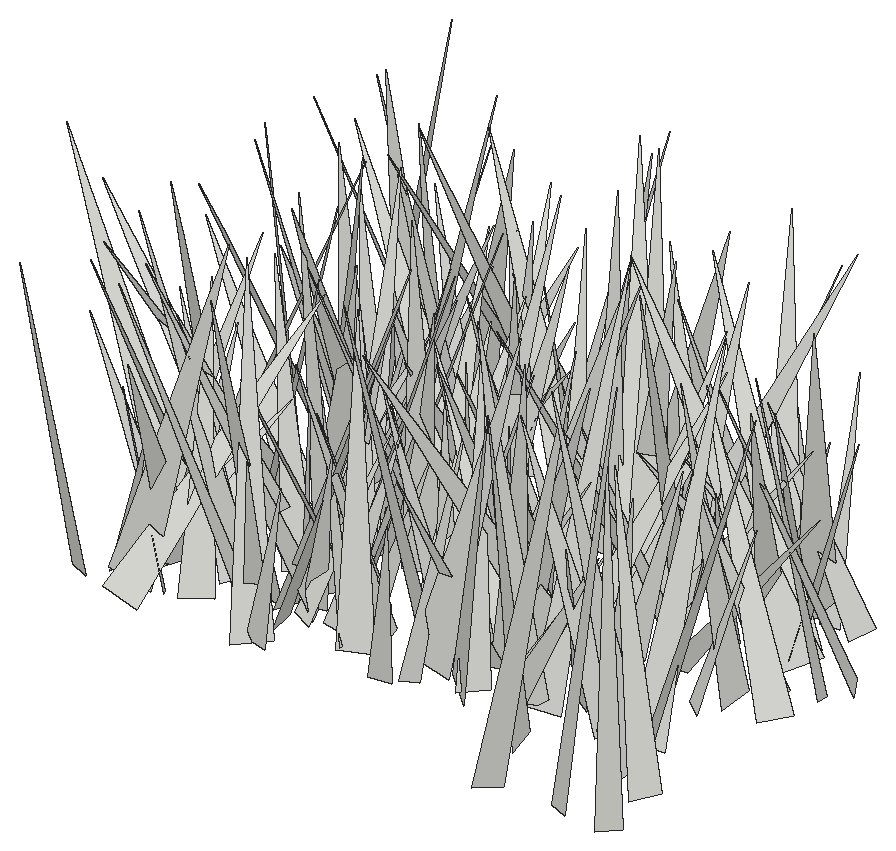
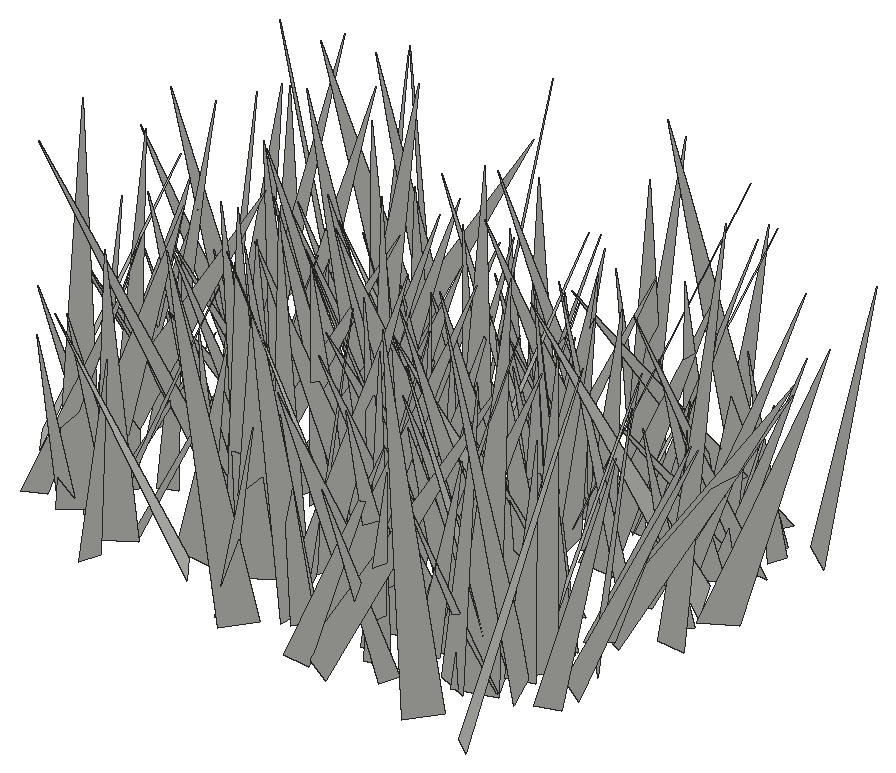
# SketchUp Ruby script. Lengths in inches.
U = 1.inch
M = Sketchup.active_model
def pt(a) = Geom::Point3d.new(a.map { |v| v * U })
def face(e, loops, mat)
  f = e.add_face(loops[0].map { |a| pt(a) })
  loops[1..].each { |l| e.add_face(l.map { |a| pt(a) }).erase! }
  f.material = f.back_material = mat if mat
  f
end
# faces: each face lists its corners as indices into pts; further lists are holes
def faces(e, pts, list, mat = nil) = list.each { |f| face(e, (f[0].is_a?(Array) ? f : [f]).map { |l| l.map { |i| pts[i] } }, mat) }
# xy, xz, yz: faces in a plane at the given z, y or x. An outline is a flat list of corners, or four numbers for a rectangle; further outlines are holes
def ring(l) = l.size == 4 ? [[l[0], l[1]], [l[2], l[1]], [l[2], l[3]], [l[0], l[3]]] : l.each_slice(2).to_a
def flat(e, list, mat, &to3) = list.each { |f| face(e, (f[0].is_a?(Array) ? f : [f]).map { |l| ring(l).map { |u, v| to3.(u, v) } }, mat) }
def xy(e, z, list, mat = nil) = flat(e, list, mat) { |x, y| [x, y, z] }
def xz(e, y, list, mat = nil) = flat(e, list, mat) { |x, z| [x, y, z] }
def yz(e, x, list, mat = nil) = flat(e, list, mat) { |y, z| [x, y, z] }
def lines(e, pts, list) = list.each { |a, b| e.add_line(pt(pts[a]), pt(pts[b])) }
# prism: a flat outline (further loops are holes) pulled along v
def prism(e, loops, v, mat = nil)
  f = face(e, loops, mat); d = Geom::Vector3d.new(v.map { |x| x * U })
  f.pushpull(f.normal.samedirection?(d) ? d.length : -d.length)
end
def box(e, o, s, mat = nil) = prism(e, [[o, [o[0] + s[0], o[1], o[2]], [o[0] + s[0], o[1] + s[1], o[2]], [o[0], o[1] + s[1], o[2]]]], [0, 0, s[2]], mat)
def at(x, y, z, deg = 0) = Geom::Transformation.translation(pt([x, y, z])) * Geom::Transformation.rotation(ORIGIN, Z_AXIS, deg.degrees)
def axes(o, x, y, z) = Geom::Transformation.new([*x, 0, *y, 0, *z, 0, *pt(o).to_a, 1])
def part(name) = M.definitions.add(name)
# library, detail: a bought-in or finely detailed component or shape, given as its bounding box
def library(name, o, s) = part(name).tap { |d| box(d.entities, o, s) }
def detail(e, o, s) = box(e.add_group.entities, o, s)
def put(e, d, t, mat = nil) = e.add_instance(d, t).tap { |i| i.material = mat if mat }
def group(e, t, mat = nil) = e.add_group.tap { |g| g.transformation = t; g.material = mat if mat }.entities
root = M.entities
c1 = part("fur_instance\#9")
p = [[0.8125,0,1.79],[0.67,-0.02,1.48],[0,-0.11,0],[0,0.11,0]]
faces(c1.entities,p,[[0,1,2,3]])
put(root,c1,axes([73.07,325.53,-27.1],[0.44262,-3.83329,1.02735],[-3.85493,-0.16968,1.02773],[0.94293,1.1057,3.71938]))
put(root,c1,axes([91.22,322.82,-27.1],[-6.67208,0.88571,0.68005],[0.61302,6.34873,-2.25421],[0.93335,2.16166,6.3419]))
put(root,c1,axes([88.92,322.85,-27.1],[4.06044,6.49572,1.60929],[6.19974,-4.35997,1.95581],[-2.5194,-0.26008,7.4065]))
put(root,c1,axes([72.28,326.6,-27.1],[3.06057,-3.28635,0.3748],[-3.27189,-3.08287,-0.31361],[-0.4851,0.05914,4.47983]))
put(root,c1,axes([78.15,326.22,-27.1],[1.46502,-3.697,0.60293],[-3.73698,-1.39797,0.50827],[0.25762,0.74531,3.94408]))
put(root,c1,axes([84.83,325.88,-27.1],[-6.1633,-1.76581,2.36846],[-1.74431,6.59751,0.37966],[2.38433,0.26209,6.40002]))
put(root,c1,axes([85.96,322.57,-27.1],[7.23662,0.86237,3.59764],[-0.54989,-7.56504,2.91946],[-3.65846,2.84288,6.67751]))
put(root,c1,axes([64.88,325.84,-27.1],[-3.28868,-4.79968,1.75844],[-5.10998,3.14053,-0.98472],[0.13097,2.01112,5.73434]))
put(root,c1,axes([72.51,326.4,-27.1],[-6.31151,-2.93767,0.11387],[-2.9284,6.25835,-0.85765],[-0.25951,0.82534,6.90866]))
put(root,c1,axes([67.33,328.63,-27.1],[4.65411,-4.15615,0.09318],[-4.0063,-4.52139,-1.56511],[-1.10988,-1.10744,6.04026]))
put(root,c1,axes([80.74,327.43,-27.1],[4.65665,4.64477,2.8893],[5.46904,-4.02795,-2.33914],[-0.10763,-3.71592,6.14709]))
put(root,c1,axes([66.7,326.41,-27.1],[0.11593,7.32982,3.76994],[7.80213,1.11829,-2.4142],[2.6581,-3.60212,6.9218]))
put(root,c1,axes([65.85,326.87,-27.1],[3.70802,-0.97097,0.29213],[-0.94384,-3.70994,-0.3508],[-0.37053,-0.26665,3.81695]))
put(root,c1,axes([90.75,325.5,-27.1],[-5.69821,2.17721,0.97614],[2.15034,5.78116,-0.34192],[1.034,-0.02439,6.0904]))
put(root,c1,axes([71.31,328.43,-27.1],[-1.28259,-7.19659,1.19017],[-7.23451,1.40948,0.72639],[0.93233,1.03678,7.27381]))
put(root,c1,axes([72.92,325.51,-27.1],[-5.4488,4.52209,1.619],[4.59694,5.6194,-0.22458],[1.39234,-0.85616,7.07731]))
put(root,c1,axes([89.22,326.78,-27.1],[-7.32255,-0.11088,1.35528],[-0.08815,7.44603,0.13288],[1.35695,-0.11461,7.32218]))
put(root,c1,axes([68.26,326.41,-27.1],[-3.16034,-1.96863,0.75138],[-2.10046,2.8354,-1.40585],[-0.16774,1.5852,3.44773]))
put(root,c1,axes([73.25,328.88,-27.1],[-6.90561,-3.33755,0.10935],[-3.32242,6.89219,0.54573],[0.33571,-0.44394,7.65042]))
put(root,c1,axes([77.89,329.3,-27.1],[-6.44031,-4.10602,1.97316],[-3.85542,6.73281,1.42663],[2.42663,-0.20036,7.50344]))
put(root,c1,axes([86.81,328.54,-27.1],[-6.00437,2.1113,1.91932],[2.55574,5.96789,1.43049],[1.26869,-2.0299,6.20191]))
put(root,c1,axes([82.78,327.9375,-27.1],[1.91277,-3.82749,0.78831],[-3.61325,-1.39793,1.9799],[1.48846,1.5251,3.7932]))
put(root,c1,axes([76.21,327.26,-27.1],[-2.20554,5.93145,2.00046],[6.2413,2.24627,0.22087],[0.47966,-1.95462,6.32437]))
put(root,c1,axes([78.94,328.03,-27.1],[1.45839,-7.20301,2.88114],[-7.56056,-0.66269,2.17028],[1.73849,3.16049,7.02141]))
put(root,c1,axes([80.76,329.47,-27.1],[-0.13118,-4.53208,0.33432],[-4.41868,0.04908,-1.06843],[-1.06148,0.35576,4.40629]))
put(root,c1,axes([71.19,327.65,-27.1],[-7.48937,-0.81173,0.36322],[-0.84224,7.4632,-0.68756],[0.28542,0.72333,7.50179]))
put(root,c1,axes([73.09,328.85,-27.1],[1.90373,-3.64825,0.45227],[-3.65968,-1.83258,0.622],[0.34793,0.68584,4.0678]))
put(root,c1,axes([69.4,326.8,-27.1],[-4.06626,4.25963,1.22614],[4.27905,4.20638,-0.4224],[1.15655,-0.5867,5.87371]))
put(root,c1,axes([76.52,328.84,-27.1],[-5.39834,-1.72938,0.70035],[-1.70183,5.44274,0.32197],[0.76486,-0.09564,5.65943]))
put(root,c1,axes([84.68,329.375,-27.1],[-1.23844,-4.00226,0.78585],[-3.84524,1.41955,1.16979],[1.36007,0.36904,4.02286]))
put(root,c1,axes([67.08,328.48,-27.1],[-4.89818,0.93846,0.55806],[1.01529,4.8584,0.74127],[0.40164,-0.83642,4.93188]))
put(root,c1,axes([82.5,328.17,-27.1],[1.50617,-3.93782,1.16858],[-3.70084,-0.76096,2.20573],[1.78207,1.74788,3.59301]))
put(root,c1,axes([83.39,328.21,-27.1],[0.00148,-6.83986,3.17541],[-7.42007,-0.56775,-1.21947],[-1.34516,3.12424,6.73027]))
put(root,c1,axes([74.7,329.66,-27.1],[-2.68226,-4.58353,0.12394],[-4.53778,2.63294,-0.83358],[-0.65781,0.52677,5.24485]))
put(root,c1,axes([72.86,327.26,-27.1],[6.72772,1.76518,0.89994],[1.69777,-6.77807,0.60273],[-1.02144,0.36032,6.92927]))
put(root,c1,axes([67.28,325.14,-27.1],[-1.44675,6.62808,0.1342],[5.91861,1.35324,-3.03008],[2.98656,0.529,6.06986]))
put(root,c1,axes([86.77,328.54,-27.1],[4.38951,-2.01268,1.547],[-2.15257,-4.58905,0.13732],[-1.34555,0.7756,4.82698]))
put(root,c1,axes([74.67,328.08,-27.1],[-0.11814,4.24138,1.60816],[4.31681,0.59918,-1.26317],[1.39308,-1.49704,4.05064]))
put(root,c1,axes([75.74,327.44,-27.1],[-4.50739,-0.00087,0.31518],[-0.09503,4.31184,-1.34718],[0.30051,1.35052,4.30136]))
put(root,c1,axes([79.03,326.79,-27.1],[-4.41847,1.33903,1.10997],[0.76139,4.21375,-2.05244],[1.56375,1.73183,4.13562]))
put(root,c1,axes([67.36,330.45,-27.1],[-2.8111,-5.64649,0.53318],[-5.64839,2.7334,-0.83291],[-0.51273,0.84565,6.25232]))
put(root,c1,axes([82.77,331.55,-27.1],[1.75618,-7.20882,1.45322],[-6.25973,-2.24953,-3.59425],[-3.85938,0.3683,6.49097]))
put(root,c1,axes([73.26,327.93,-27.1],[1.23248,3.89294,0.26564],[3.83774,-1.15903,-0.82034],[0.70519,-0.49622,4.00013]))
put(root,c1,axes([78.68,329.61,-27.1],[-5.18821,0.426,1.12668],[0.56814,5.25845,0.62796],[1.06213,-0.73187,5.16766]))
put(root,c1,axes([81.22,327.67,-27.1],[-5.70691,2.72816,1.15825],[2.57005,5.80682,-1.01437],[1.47624,0.43731,6.24361]))
put(root,c1,axes([69.62,328.71,-27.1],[-4.99004,2.24313,0.58277],[2.2784,5.00139,0.2583],[0.42444,-0.4756,5.46492]))
put(root,c1,axes([75.4375,330.22,-27.1],[-3.54687,-2.63553,0.56126],[-2.61948,3.58991,0.30355],[0.63194,0.08835,4.40842]))
put(root,c1,axes([66.41,327.62,-27.1],[-0.23722,4.19444,0.05409],[3.55446,0.22976,-2.22834],[2.22756,0.08005,3.56147]))
put(root,c1,axes([68.89,328.75,-27.1],[-3.32365,-1.7064,1.24939],[-2.04417,3.18881,-1.08271],[0.54234,1.56176,3.57578]))
put(root,c1,axes([70.47,331.37,-27.1],[2.04194,-5.37013,1.21962],[-4.97283,-2.35693,-2.05211],[-2.36574,0.31918,5.36625]))
put(root,c1,axes([75.47,328.96,-27.1],[3.08965,-1.86478,1.07968],[-2.12915,-2.93231,1.02827],[-0.33144,1.45368,3.45919]))
put(root,c1,axes([80.73,330.3,-27.1],[5.91489,-2.56905,1.81184],[-2.61095,-6.16477,-0.21752],[-1.75092,0.51416,6.44505]))
put(root,c1,axes([80.55,330.73,-27.1],[5.68552,-4.38043,0.51347],[-4.40819,-5.61738,0.88871],[0.14016,1.01677,7.12204]))
put(root,c1,axes([71.83,329.9,-27.1],[1.95949,2.80373,1.45551],[3.04239,-2.136,0.01872],[-0.85045,-1.18135,3.42055]))
put(root,c1,axes([66.7,329.45,-27.1],[1.07751,-3.9043,2.33703],[-4.53898,-0.75293,0.83488],[0.32078,2.46086,3.96327]))
put(root,c1,axes([72.22,328.33,-27.1],[6.79493,0.95964,1.40947],[0.56386,-6.72962,1.86359],[-1.60922,1.6941,6.60447]))
put(root,c1,axes([72.9,330.04,-27.1],[4.01633,-1.15722,1.23996],[-1.33038,-4.12648,0.45808],[-1.05202,0.80037,4.15454]))
put(root,c1,axes([65.91,328.12,-27.1],[1.29367,6.30142,0.29631],[6.29029,-1.26564,-0.54746],[0.47747,-0.39942,6.4095]))
put(root,c1,axes([88.75,328.15,-27.1],[5.94248,2.0649,1.47313],[1.51819,-5.90154,2.14801],[-2.032,1.62942,5.91295]))
put(root,c1,axes([88.48,328.4,-27.1],[0.44326,7.59594,0.73525],[7.62112,-0.4789,0.35297],[-0.39679,-0.71255,7.60067]))
put(root,c1,axes([73.14,330.38,-27.1],[6.72571,2.73267,0.89443],[2.78268,-6.75899,-0.27437],[-0.72399,-0.59256,7.25447]))
put(root,c1,axes([79.02,331.21,-27.1],[3.3459,3.39415,0.39754],[3.18536,-2.89609,-2.08314],[1.23764,-1.72213,4.2867]))
put(root,c1,axes([77.96,329.58,-27.1],[5.23362,2.8594,0.35445],[2.818,-5.23298,0.60609],[-0.60055,0.36375,5.93293]))
put(root,c1,axes([81.11,330.34,-27.1],[-3.6214,4.75768,0.36392],[4.63089,3.39426,1.70771],[-1.15013,-1.31374,5.73008]))
put(root,c1,axes([80.07,332.96,-27.1],[0.31088,-6.10314,0.84199],[-6.04835,-0.46277,-1.12122],[-1.17245,0.76905,6.00731]))
put(root,c1,axes([71.03,330.5625,-27.1],[-1.86081,5.49202,1.44787],[5.66351,1.67938,0.90859],[-0.42807,-1.65488,5.72707]))
put(root,c1,axes([77.08,331.4,-27.1],[4.20297,-1.11156,0.80651],[-1.18233,-4.24977,0.30429],[-0.69867,0.5049,4.33681]))
put(root,c1,axes([84.1,328.08,-27.1],[1.42623,8.08681,0.06748],[7.92603,-1.41139,1.61901],[-1.60595,0.21606,8.05043]))
put(root,c1,axes([64.93,334.06,-27.1],[-2.27672,-7.40144,1.23154],[-7.29478,2.48469,1.44709],[1.75622,0.72557,7.60728]))
put(root,c1,axes([75.4375,333.28,-27.1],[-5.5722,-4.07145,0.43281],[-4.071,5.58734,0.1482],[0.43699,0.13539,6.89957]))
put(root,c1,axes([76.88,331.82,-27.1],[4.42426,3.38365,0.88099],[3.49585,-4.30744,-1.01209],[-0.06566,-1.34021,5.47712]))
put(root,c1,axes([64.62,331.75,-27.1],[-5.80896,4.38047,0.69826],[4.41604,5.60261,1.59041],[-0.41794,-1.68592,7.09952]))
put(root,c1,axes([76.01,332.125,-27.1],[-2.1087,-2.96786,0.97974],[-3.12443,1.97245,-0.74971],[-0.07759,1.23123,3.56269]))
put(root,c1,axes([72.08,330.91,-27.1],[-6.95078,-0.2098,1.40903],[-0.48679,6.94525,-1.36721],[1.33881,1.43604,6.81821]))
put(root,c1,axes([88.07,331.55,-27.1],[2.28219,3.09258,0.57784],[3.14608,-2.24088,-0.43237],[0.01087,-0.72161,3.81909]))
put(root,c1,axes([88.875,332.92,-27.1],[-6.33484,-0.15602,2.15214],[0.09289,6.64883,0.75543],[2.15578,-0.74496,6.29157]))
put(root,c1,axes([80.07,334.48,-27.1],[-0.6438,-6.00502,0.1729],[-5.98541,0.62626,-0.53591],[-0.51472,0.22839,6.0156]))
put(root,c1,axes([67.98,332.39,-27.1],[-5.05806,4.73106,0.08976],[4.36112,4.60989,2.7757],[-1.83619,-2.08349,6.34527]))
put(root,c1,axes([65.36,332.8,-27.1],[1.8239,-3.22944,0.77362],[-3.28665,-1.6292,0.94764],[0.47508,1.1273,3.58579]))
put(root,c1,axes([77.46,332.22,-27.1],[-4.422,-0.95671,1.75223],[-1.16644,4.69405,-0.38074],[1.6202,0.76828,4.50826]))
put(root,c1,axes([79.42,331.88,-27.1],[2.90611,1.79436,1.69144],[1.585,-3.36196,0.84331],[-1.88904,-0.06039,3.30969]))
put(root,c1,axes([74.49,333.29,-27.1],[2.05152,-6.96349,2.48946],[-7.36809,-2.14532,0.07104],[-0.63146,2.40909,7.25905]))
put(root,c1,axes([72.55,333.27,-27.1],[3.14021,-1.95272,0.11029],[-1.95573,-3.13292,0.21476],[0.01996,0.24059,3.6916]))
put(root,c1,axes([73.45,334.22,-27.1],[0.26156,-6.27199,1.2943],[-6.21893,0.06053,1.55008],[1.52905,1.31908,6.08306]))
put(root,c1,axes([75.52,333.23,-27.1],[2.21811,-2.97156,1.30139],[-3.14682,-2.35396,-0.01147],[-0.78819,1.03561,3.7081]))
put(root,c1,axes([67.13,334.91,-27.1],[-0.73144,-5.99959,0.26703],[-5.39662,0.53861,-2.681],[-2.63493,0.56233,5.41685]))
put(root,c1,axes([89.89,334.05,-27.1],[-4.18916,1.41328,1.44955],[1.84035,4.04661,1.3732],[0.84361,-1.80976,4.20247]))
put(root,c1,axes([84,333.22,-27.1],[1.31447,-3.85278,1.5031],[-4.0825,-0.95693,1.11736],[0.66058,1.75255,3.91449]))
put(root,c1,axes([70.5,333.52,-27.1],[2.46707,-3.42013,1.11602],[-3.59628,-2.30764,0.87798],[0.09798,1.4166,4.12467]))
put(root,c1,axes([71.97,333.03,-27.1],[2.76185,-3.07557,2.49035],[-3.57907,-3.23702,-0.02845],[-1.68858,1.83068,4.13354]))
put(root,c1,axes([90.82,332.74,-27.1],[-3.78677,4.88862,0.77178],[4.90876,3.58599,1.37062],[-0.63111,-1.44081,6.0299]))
put(root,c1,axes([72.1875,334.22,-27.1],[2.06201,-3.51619,0.27094],[-3.44771,-1.94389,1.0117],[0.74186,0.73932,3.94867]))
put(root,c1,axes([65.99,330.82,-27.1],[6.85876,3.23862,0.41321],[3.02392,-6.66397,2.03701],[-1.23097,1.67477,7.30628]))
put(root,c1,axes([77.49,332.42,-27.1],[5.50822,-3.47682,2.75588],[-4.25576,-5.38219,1.71589],[-1.25366,2.99458,6.28367]))
put(root,c1,axes([67.02,333.6875,-27.1],[6.14666,2.4589,1.36982],[2.59506,-6.2248,-0.47069],[-1.09008,-0.95377,6.60349]))
put(root,c1,axes([83.87,335.44,-27.1],[-4.5248,-1.88356,0.71077],[-1.69814,4.51006,1.14127],[1.08134,-0.799,4.76646]))
put(root,c1,axes([85.78,333.42,-27.1],[3.92135,-2.35365,0.03406],[-2.05535,-3.39138,2.27856],[1.14733,1.96892,3.96545]))
put(root,c1,axes([77.99,330.71,-27.1],[-7.05102,3.6652,1.50452],[2.87345,6.84526,-3.20935],[2.72774,2.26338,7.26985]))
put(root,c1,axes([75.72,332.33,-27.1],[-0.62554,4.99616,0.12365],[4.99768,0.62512,0.02455],[-0.009,-0.12574,5.03511]))
put(root,c1,axes([83.17,336.02,-27.1],[-1.63485,-6.2778,0.46595],[-5.97391,1.39539,-2.16005],[-1.98499,0.97094,6.117]))
put(root,c1,axes([81.95,332.625,-27.1],[1.01067,5.88602,0.15693],[5.68933,-0.93518,-1.56469],[1.51703,-0.41415,5.76354]))
put(root,c1,axes([70.53,335.16,-27.1],[4.49175,-3.99144,0.42922],[-3.97143,-4.32409,1.3497],[0.58618,1.28931,5.8554]))
put(root,c1,axes([76.25,336.04,-27.1],[6.0824,-3.06076,1.36011],[-2.97573,-6.23245,-0.71791],[-1.53726,-0.04598,6.77115]))
put(root,c1,axes([83.47,336.77,-27.1],[-6.68782,-2.79113,3.18251],[-2.04813,7.34131,2.13449],[3.70459,-0.98003,6.92541]))
put(root,c1,axes([68.82,337.78,-27.1],[1.6119,-7.35068,0.1441],[-7.34568,-1.61634,-0.28263],[-0.30696,0.08011,7.52003]))
put(root,c1,axes([85.86,336.31,-27.1],[0.30074,-4.21199,0.28121],[-4.14735,-0.24225,0.80695],[0.78703,0.33293,4.14489]))
put(root,c1,axes([74.26,337.84,-27.1],[4.06405,-3.6671,0.18626],[-3.28339,-3.75381,-2.26428],[-1.64366,-1.56845,4.98369]))
put(root,c1,axes([91.61,336.26,-27.1],[-5.39414,-3.77764,0.22745],[-3.78403,5.38986,-0.22257],[0.05845,0.31282,6.58162]))
put(root,c1,axes([87.12,337.3,-27.1],[6.03542,-2.39463,0.80521],[-2.12324,-5.9379,-1.74415],[-1.3691,-1.34759,6.25448]))
put(root,c1,axes([84.47,335.59,-27.1],[3.53808,2.09554,0.91862],[2.27584,-3.39762,-1.01485],[-0.23603,-1.34836,3.98489]))
put(root,c1,axes([72.92,332.33,-27.1],[5.4592,3.52611,0.65952],[3.05756,-5.20187,2.50265],[-1.87611,1.78282,5.99776]))
put(root,c1,axes([68.83,334.35,-27.1],[1.67584,3.97009,0.12724],[3.80521,-1.56498,-1.28741],[1.13936,-0.61275,4.1125]))
put(root,c1,axes([77.63,335.45,-27.1],[2.98572,-5.88102,1.99527],[-6.13329,-2.44486,1.97166],[0.97482,2.63026,6.29392]))
put(root,c1,axes([81.78,333.04,-27.1],[-2.11402,4.56513,0.60738],[3.84978,2.11854,-2.52378],[2.52756,0.59144,4.35202]))
put(root,c1,axes([67.08,335.4,-27.1],[-4.48303,2.72425,0.35571],[2.72908,4.33728,1.17718],[-0.3165,-1.18832,5.11208]))
put(root,c1,axes([67.66,336.71,-27.1],[0.9975,-5.62203,0.93729],[-5.55991,-0.75041,1.41599],[1.25425,1.14473,5.53148]))
put(root,c1,axes([72.56,335.22,-27.1],[3.74419,-3.98525,0.35569],[-3.51637,-3.04515,2.89653],[1.90889,2.20738,4.63803]))
put(root,c1,axes([81.13,333.12,-27.1],[-6.61706,2.95045,0.41304],[2.75432,6.44194,-1.89112],[1.13554,1.56763,6.99387]))
put(root,c1,axes([91.19,334.93,-27.1],[-5.46466,-2.11839,0.66349],[-2.21236,5.05235,-2.09036],[-0.18243,2.18553,5.47545]))
put(root,c1,axes([77.83,334.73,-27.1],[6.41211,-0.61612,1.30158],[-0.93497,-6.2989,1.62436],[-1.09524,1.77006,6.23347]))
put(root,c1,axes([70.88,334.27,-27.1],[-0.70792,6.63222,0.94241],[6.69223,0.65809,0.39581],[-0.29764,-0.97786,6.65814]))
put(root,c1,axes([77.05,336.51,-27.1],[-4.90354,-1.85753,0.89414],[-1.8937,4.97041,-0.05944],[0.81474,0.37312,5.24324]))
put(root,c1,axes([83.23,335.88,-27.1],[3.04424,4.32162,0.01521],[3.85535,-2.70735,-2.39804],[1.95268,-1.39208,4.71097]))
put(root,c1,axes([89.12,336.36,-27.1],[-4.49913,6.58347,1.21187],[6.27218,3.63575,3.53468],[-2.33889,-2.91414,7.14775]))
put(root,c1,axes([81.84,334.91,-27.1],[0.68062,5.93772,0.86921],[5.89172,-0.495,-1.23203],[1.14003,-0.98679,5.84823]))
put(root,c1,axes([67.07,337.3,-27.1],[6.76883,1.43904,1.95286],[1.74836,-6.90673,-0.9705],[-1.68159,-1.38844,6.85171]))
put(root,c1,axes([73.89,334.82,-27.1],[-1.59492,4.69203,0.53683],[4.53057,1.68008,-1.22409],[1.33316,-0.09626,4.80214]))
put(root,c1,axes([68.02,337.55,-27.1],[-5.59539,-3.44886,0.89561],[-3.54081,5.56848,-0.67808],[0.39927,1.05,6.53783]))
put(root,c1,axes([76.33,337.62,-27.1],[-3.68845,0.83243,0.84341],[0.99836,3.66829,0.74556],[0.6384,-0.92717,3.70698]))
put(root,c1,axes([84.67,339.625,-27.1],[-4.21387,-1.59887,0.24339],[-1.27519,3.70248,2.24451],[0.99474,-2.02671,3.90836]))
put(root,c1,axes([83.42,336.08,-27.1],[-1.23701,6.48468,1.94316],[6.59867,1.59608,-1.12573],[1.51147,-1.6609,6.50492]))
put(root,c1,axes([86.75,339.47,-27.1],[-1.94792,-5.41513,0.85515],[-5.11405,2.12183,1.78705],[1.97517,0.15336,5.47032]))
put(root,c1,axes([66.1875,336.7,-27.1],[-4.69579,-3.74143,2.09942],[-4.25802,4.44495,-1.60248],[0.52452,2.58851,5.78625]))
put(root,c1,axes([65.65,338.75,-27.1],[-2.53227,-4.93937,0.36335],[-4.86121,2.40071,-1.24381],[-0.94765,0.88376,5.4095]))
put(root,c1,axes([87.44,339.37,-27.1],[4.02071,-6.30995,0.86141],[-6.36147,-4.02715,0.19326],[-0.29869,0.83076,7.47959]))
put(root,c1,axes([88.56,336.65,-27.1],[4.03699,1.00135,1.00845],[0.75439,-4.0837,1.03503],[-1.2044,0.79854,4.02849]))
put(root,c1,axes([77.62,338.45,-27.1],[-4.6895,-2.45579,1.69505],[-2.43913,4.97359,0.45768],[1.71894,0.35769,5.27378]))
put(root,c1,axes([88.63,336.83,-27.1],[-6.09178,4.42452,0.24879],[4.41982,6.03543,0.88707],[-0.32169,-0.86331,7.47659]))
put(root,c1,axes([86.35,339.97,-27.1],[-4.14982,-0.72477,0.23143],[-0.53834,3.70403,1.94686],[0.53763,-1.88541,3.73578]))
put(root,c1,axes([82.15,338.15,-27.1],[-3.43259,1.11019,2.13702],[1.24058,4.00441,-0.08763],[2.06406,-0.56053,3.60659]))
put(root,c1,axes([67.32,338.55,-27.1],[-4.56803,3.68378,2.77525],[4.20348,4.93276,0.37129],[1.89817,-2.05836,5.85656]))
put(root,c1,axes([68.46,337.73,-27.1],[2.21445,2.95218,0.72503],[3.03203,-2.20951,-0.26401],[-0.21871,-0.73996,3.68096]))
put(root,c1,axes([70.8,339.46,-27.1],[0.6809,-4.24063,0.83858],[-4.19337,-0.85411,-0.91428],[-1.04966,0.66131,4.19651]))
put(root,c1,axes([82.3125,336.6,-27.1],[2.96543,7.80813,0.73471],[7.53088,-2.61577,-2.59693],[2.18919,-1.57838,7.9383]))
put(root,c1,axes([65.54,340.24,-27.1],[3.46395,-3.11936,0.86631],[-2.7787,-3.51575,-1.54862],[-1.66124,-0.62369,4.39672]))
put(root,c1,axes([79.36,339.33,-27.1],[2.15737,-6.51602,1.69287],[-6.69271,-1.88316,1.28061],[0.7294,1.99342,6.74336]))
put(root,c1,axes([78.76,338.29,-27.1],[-0.16128,6.84934,2.86842],[7.42417,0.20732,-0.07764],[0.15166,-2.86546,6.8508]))
put(root,c1,axes([72.83,336.35,-27.1],[-4.26385,3.34064,0.29483],[3.15748,4.15963,-1.468],[1.13011,0.98225,5.21395]))
put(root,c1,axes([89.44,339.41,-27.1],[-4.32688,2.05759,1.06704],[2.30248,4.07514,1.47851],[0.2661,-1.80382,4.55737]))
put(root,c1,axes([78.07,337.97,-27.1],[-7.19785,3.45896,0.52945],[3.49375,7.17168,0.64382],[0.19618,-0.81015,7.95983]))
put(root,c1,axes([70.93,336.17,-27.1],[7.1916,2.06862,2.54607],[1.20326,-7.37063,2.58975],[-3.05186,1.96861,7.0208]))
put(root,c1,axes([86.28,338.52,-27.1],[3.72364,-1.08643,0.80362],[-1.21362,-3.72465,0.58799],[-0.59435,0.79892,3.83407]))
put(root,c1,axes([72.51,338.23,-27.1],[-5.71185,4.45959,0.23835],[4.39877,5.55102,1.55146],[-0.77178,-1.36683,7.07857]))
put(root,c1,axes([73.46,339.5625,-27.1],[0.07384,-6.03784,2.03973],[-6.28438,0.27016,1.02718],[1.05955,2.02311,5.95028]))
put(root,c1,axes([86.18,339.14,-27.1],[-5.88175,-1.50758,0.15009],[-1.51502,5.85044,-0.60606],[-0.00586,0.62434,6.04156]))
put(root,c1,axes([72.93,338.21,-27.1],[-7.75285,-2.01113,0.68817],[-2.11722,7.53738,-1.82488],[0.1887,1.94117,7.79879]))
put(root,c1,axes([80.83,338.03,-27.1],[-1.87564,7.62096,1.95831],[7.8685,1.80971,0.49369],[-0.027,-2.0194,7.83284]))
put(root,c1,axes([68.62,338.71,-27.1],[4.54931,-2.96003,1.24819],[-3.21199,-4.22741,1.68171],[-0.05363,2.09362,5.16041]))
put(root,c1,axes([71.14,338.75,-27.1],[0.71966,5.69009,1.64056],[5.43341,0.02279,-2.46251],[2.35511,-1.79132,5.17987]))
put(root,c1,axes([76.89,337,-27.1],[-5.00496,1.9066,1.35129],[1.19771,4.83542,-2.3864],[2.00664,1.8693,4.79477]))
put(root,c1,axes([77.54,336.37,-27.1],[5.51307,6.12337,0.96272],[5.81555,-5.55551,2.03274],[-2.14519,0.67601,7.98483]))
put(root,c1,axes([67.55,339.27,-27.1],[1.73924,-4.25815,2.51532],[-4.74882,-2.1825,-0.41111],[-1.38108,2.14207,4.58125]))
put(root,c1,axes([80.45,337.91,-27.1],[-5.1988,6.07272,1.14347],[6.1224,5.26442,-0.12263],[0.83765,-0.78798,7.99315]))
put(root,c1,axes([68.25,340.98,-27.1],[2.83404,-7.21043,2.36501],[-7.48804,-3.06648,-0.37599],[-1.22999,2.05469,7.73827]))
put(root,c1,axes([74.44,342.21,-27.1],[-0.7633,-7.78268,1.04828],[-7.63293,0.4877,-1.93706],[-1.84592,1.20152,7.57632]))
put(root,c1,axes([72.22,341.52,-27.1],[-0.22733,-5.68785,1.31588],[-5.73337,0.46581,1.02292],[1.10075,1.2515,5.59972]))
put(root,c1,axes([76.11,340.86,-27.1],[3.13443,-2.25979,0.73802],[-2.32723,-3.16608,0.18952],[-0.4851,0.5876,3.85946]))
put(root,c1,axes([67.9375,339.78,-27.1],[5.69643,3.12279,1.00252],[3.16084,-5.76326,-0.00802],[-0.87518,-0.48903,6.49623]))
put(root,c1,axes([88.14,339.16,-27.1],[0.35019,4.61175,0.40741],[4.56098,-0.41379,0.76359],[-0.79477,-0.34263,4.56155]))
put(root,c1,axes([73.7,338.73,-27.1],[-2.14385,5.53708,0.23418],[5.53457,2.15208,-0.21752],[0.2875,-0.13964,5.93364]))
put(root,c1,axes([82.11,339.61,-27.1],[-1.56415,5.71782,0.81541],[5.62888,1.31989,1.54221],[-1.29382,-1.17019,5.72377]))
put(root,c1,axes([76.65,340.4375,-27.1],[7.07212,-1.1156,2.41076],[-1.38462,-7.39913,0.63784],[-2.26697,1.03896,7.1311]))
put(root,c1,axes([69.17,341.1,-27.1],[1.62899,5.48386,2.82302],[6.01922,-2.05055,0.50999],[-1.34582,-2.53344,5.69792]))
put(root,c1,axes([71.02,340.3125,-27.1],[-4.64621,2.31988,0.55706],[2.32982,4.67441,-0.03457],[0.51391,-0.21773,5.19306]))
put(root,c1,axes([73.86,343,-27.1],[-2.5504,-6.61055,0.06946],[-6.29815,2.40698,-2.17909],[-2.00934,0.84606,6.74207]))
put(root,c1,axes([67.83,340.59,-27.1],[1.33461,3.80482,0.72121],[3.71713,-1.04467,-1.36733],[1.08616,-1.09999,3.79319]))
put(root,c1,axes([67.06,339.76,-27.1],[7.33246,2.99097,2.42144],[2.72494,-7.71469,1.27771],[-2.71735,0.33456,7.81527]))
put(root,c1,axes([66.19,344.25,-27.1],[-4.76858,-5.56642,0.65425],[-5.40433,4.79429,1.40014],[1.48534,-0.42682,7.19472]))
put(root,c1,axes([84.95,340.32,-27.1],[-3.82919,5.78151,1.38736],[5.88668,3.91838,-0.08139],[0.83523,-1.11076,6.93412]))
put(root,c1,axes([72.9,340.89,-27.1],[-1.18349,4.29439,0.91251],[4.36217,1.04349,0.74676],[-0.49586,-1.06979,4.39144]))
put(root,c1,axes([77.81,342.36,-27.1],[4.01839,-5.64573,1.18023],[-5.73753,-3.76564,1.52164],[0.58986,1.83314,6.76065]))
put(root,c1,axes([74.61,343.1,-27.1],[1.33499,-4.14938,1.03511],[-3.92508,-1.61935,-1.42916],[-1.69781,0.48101,4.1179]))
put(root,c1,axes([78.79,342.01,-27.1],[-3.8802,0.07929,1.10053],[0.11582,4.03064,0.11798],[1.09728,-0.14508,3.87922]))
put(root,c1,axes([71.18,342.17,-27.1],[2.09245,-2.98815,0.44058],[-2.87886,-1.81085,1.39087],[0.91397,1.13723,3.37237]))
put(root,c1,axes([84.93,341.88,-27.1],[-3.91308,1.33626,1.31278],[1.41439,4.10109,0.04154],[1.2282,-0.46546,4.13474]))
put(root,c1,axes([68.6,343.43,-27.1],[5.57249,-4.36069,0.56036],[-4.38496,-5.5781,0.19774],[-0.31889,0.50141,7.07313]))
put(root,c1,axes([81.72,340.35,-27.1],[5.03516,3.5658,0.22039],[3.50469,-5.00395,0.89105],[-0.69327,0.6016,6.10523]))
